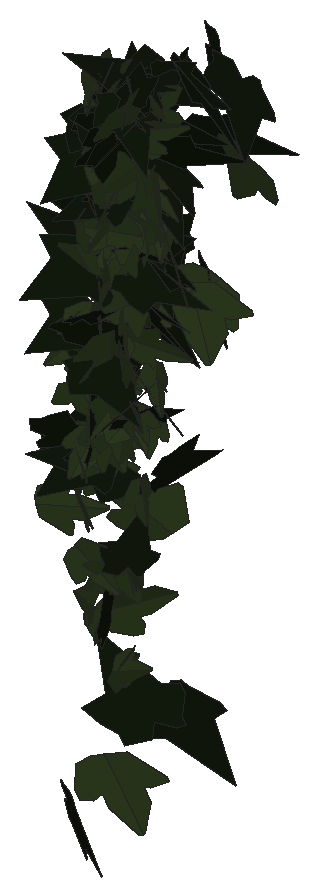
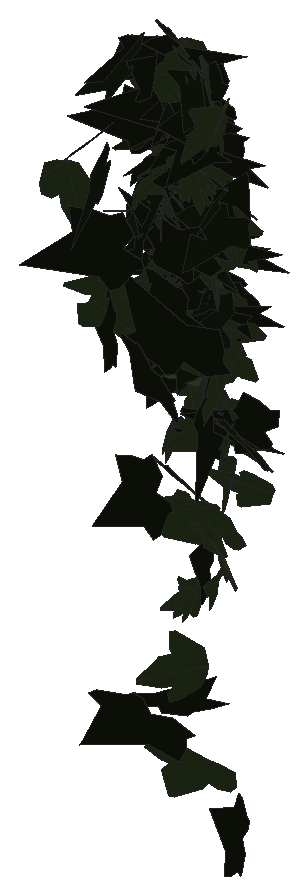
# SketchUp Ruby script. Lengths in inches.
U = 1.inch
M = Sketchup.active_model
def pt(a) = Geom::Point3d.new(a.map { |v| v * U })
def face(e, loops, mat)
  f = e.add_face(loops[0].map { |a| pt(a) })
  loops[1..].each { |l| e.add_face(l.map { |a| pt(a) }).erase! }
  f.material = f.back_material = mat if mat
  f
end
# faces: each face lists its corners as indices into pts; further lists are holes
def faces(e, pts, list, mat = nil) = list.each { |f| face(e, (f[0].is_a?(Array) ? f : [f]).map { |l| l.map { |i| pts[i] } }, mat) }
# xy, xz, yz: faces in a plane at the given z, y or x. An outline is a flat list of corners, or four numbers for a rectangle; further outlines are holes
def ring(l) = l.size == 4 ? [[l[0], l[1]], [l[2], l[1]], [l[2], l[3]], [l[0], l[3]]] : l.each_slice(2).to_a
def flat(e, list, mat, &to3) = list.each { |f| face(e, (f[0].is_a?(Array) ? f : [f]).map { |l| ring(l).map { |u, v| to3.(u, v) } }, mat) }
def xy(e, z, list, mat = nil) = flat(e, list, mat) { |x, y| [x, y, z] }
def xz(e, y, list, mat = nil) = flat(e, list, mat) { |x, z| [x, y, z] }
def yz(e, x, list, mat = nil) = flat(e, list, mat) { |y, z| [x, y, z] }
def lines(e, pts, list) = list.each { |a, b| e.add_line(pt(pts[a]), pt(pts[b])) }
# prism: a flat outline (further loops are holes) pulled along v
def prism(e, loops, v, mat = nil)
  f = face(e, loops, mat); d = Geom::Vector3d.new(v.map { |x| x * U })
  f.pushpull(f.normal.samedirection?(d) ? d.length : -d.length)
end
def box(e, o, s, mat = nil) = prism(e, [[o, [o[0] + s[0], o[1], o[2]], [o[0] + s[0], o[1] + s[1], o[2]], [o[0], o[1] + s[1], o[2]]]], [0, 0, s[2]], mat)
def at(x, y, z, deg = 0) = Geom::Transformation.translation(pt([x, y, z])) * Geom::Transformation.rotation(ORIGIN, Z_AXIS, deg.degrees)
def axes(o, x, y, z) = Geom::Transformation.new([*x, 0, *y, 0, *z, 0, *pt(o).to_a, 1])
def part(name) = M.definitions.add(name)
# library, detail: a bought-in or finely detailed component or shape, given as its bounding box
def library(name, o, s) = part(name).tap { |d| box(d.entities, o, s) }
def detail(e, o, s) = box(e.add_group.entities, o, s)
def put(e, d, t, mat = nil) = e.add_instance(d, t).tap { |i| i.material = mat if mat }
def group(e, t, mat = nil) = e.add_group.tap { |g| g.transformation = t; g.material = mat if mat }.entities
root = M.entities
M.materials.add("1026 AP 7946 SUNNY SIDE UP").color = [254, 231, 186]
M.materials.add("efeu1").color = [18, 25, 13]
M.materials.add("efeu2").color = [43, 57, 29]
c1 = part("ivyleaf_10")
p = [[0,0.5,-0.03],[-0.0625,2.02,-0.43],[-0.19,2.01,-0.46],[-0.54,1.05,-0.29],[-0.52,0.625,-0.18],[-0.83,0.76,-0.28],
  [-1.16,0.64,-0.33],[-1.15,0.33,-0.24],[-0.77,-0.39,0.02],[-0.3,-0.51,0.16],[0.04,-0.48,0.23],[-0.02,2.01,-0.4375],
  [-0.06,2.01,-0.43],[0.04,-0.49,0.23],[0.67,-0.49,0.14],[1.38,0.36,-0.2],[1.375,0.51,-0.24],[0.81,0.65,-0.19],
  [0.62,0.59,-0.15],[0.6,1.09,-0.28],[0.5,1.23,-0.31]]
faces(c1.entities,p,[[0,1,2,3,4,5,6,7,8,9,10],[11,12,0,13,14,15,16,17,18,19,20]],"efeu2")
c2 = part("ivyleaf_9")
p = [[1.54,2.16,1.25],[1.36,2.04,1.19],[-0.21,0.99,0.68],[-0.71,1.11,0.82],[-0.85,0.86,0.67],[-0.8,0.17,0.21],
  [-0.9,-0.01,0.1],[-0.67,-0.16,-0.02],[-0.08,-0.08,-0.05],[-0.03,-0.6,-0.4],[0.65,-0.88,-0.66],[0.83,-0.6,-0.49],
  [1.29,-0.42,-0.43],[1.8125,-0.07,-0.26],[1.21,0.44,0.15]]
faces(c2.entities,p,[[0,1,2,3,4,5,6,7,8,9,10,11,12,13,14]],"efeu1")
put(root,c1,axes([138.06,210.26,263.38],[0.1291,0.1731,-0.15782],[-0.14397,-0.12604,-0.19675],[-0.33485,0.12093,0.02375]),"1026 AP 7946 SUNNY SIDE UP")
put(root,c1,axes([137.23,210.13,261.82],[0.09734,-0.04348,-0.24254],[0.37472,0.03179,0.05875],[0.03186,-0.24111,0.05]),"1026 AP 7946 SUNNY SIDE UP")
put(root,c1,axes([138.36,210.2,263.44],[-0.32079,0.0153,-0.08144],[0.11047,-0.07182,-0.20131],[-0.06213,-0.2067,0.06255]),"1026 AP 7946 SUNNY SIDE UP")
put(root,c1,axes([138.26,210.23,265.55],[0.316,-0.15134,0.01152],[-0.00357,-0.02297,-0.25851],[0.23869,0.20001,-0.01912]),"1026 AP 7946 SUNNY SIDE UP")
put(root,c1,axes([137.63,210.17,263.5],[-0.23237,-0.14034,-0.09498],[0.17288,0.01065,-0.19993],[0.19866,-0.17343,0.06289]),"1026 AP 7946 SUNNY SIDE UP")
put(root,c2,axes([137.8,210.15,264.41],[0.16591,0.16497,-0.14641],[-0.09865,-0.12928,-0.20201],[-0.32886,0.12201,-0.01327]),"1026 AP 7946 SUNNY SIDE UP")
put(root,c2,axes([138.24,210.26,267.47],[0.00262,-0.25337,-0.06246],[0.00721,0.05921,-0.26063],[0.40906,0.00058,0.005]),"1026 AP 7946 SUNNY SIDE UP")
put(root,c1,axes([138.39,210.18,266.7],[-0.31364,0.01889,0.14931],[-0.22955,-0.03335,-0.20284],[0.00709,-0.24423,0.03778]),"1026 AP 7946 SUNNY SIDE UP")
put(root,c2,axes([137.88,210.22,263.87],[-0.03443,-0.1949,-0.15408],[0.17512,0.12485,-0.18504],[0.34315,-0.08327,0.07897]),"1026 AP 7946 SUNNY SIDE UP")
put(root,c1,axes([138.36,210.12,267.53],[-0.09058,-0.29287,-0.1462],[0.06632,0.13448,-0.30637],[0.50626,-0.07002,0.01398]),"1026 AP 7946 SUNNY SIDE UP")
put(root,c2,axes([137.79,210.29,262.58],[-0.42238,0.00458,-0.0159],[0.0235,-0.02618,-0.27564],[-0.00953,-0.26779,0.0251]),"1026 AP 7946 SUNNY SIDE UP")
put(root,c1,axes([137.73,210.27,262.8],[0.19876,0.17393,-0.1307],[-0.11112,-0.10666,-0.22208],[-0.32073,0.14474,-0.00405]),"1026 AP 7946 SUNNY SIDE UP")
put(root,c1,axes([138,210.2,262.97],[-0.30622,-0.07233,-0.06685],[0.11611,-0.01707,-0.21014],[0.09865,-0.20443,0.03984]),"1026 AP 7946 SUNNY SIDE UP")
put(root,c1,axes([138.31,210.06,259.99],[-0.02923,-0.06515,-0.21105],[0.14664,0.18242,-0.06754],[0.30396,-0.09427,0.01229]),"1026 AP 7946 SUNNY SIDE UP")
put(root,c2,axes([138.36,209.96,263.46],[0.0629,0.24625,0.17947],[0.05374,0.16948,-0.25596],[-0.46998,0.05234,-0.00525]),"1026 AP 7946 SUNNY SIDE UP")
put(root,c2,axes([137.6875,210.39,265.08],[-0.35934,-0.13219,0.12933],[-0.15226,-0.08395,-0.27154],[0.24383,-0.24724,0.02103]),"1026 AP 7946 SUNNY SIDE UP")
put(root,c2,axes([138.44,210.07,261.45],[-0.30501,0.14579,0.00188],[0.01738,0.01306,0.24944],[0.22858,0.19354,-0.01646]),"1026 AP 7946 SUNNY SIDE UP")
put(root,c1,axes([138.07,210.1,265.15],[0.08744,-0.14076,-0.18635],[-0.08457,0.17208,-0.15466],[0.34931,0.0769,0.0092]),"1026 AP 7946 SUNNY SIDE UP")
put(root,c1,axes([137.52,210.375,264.11],[0.14013,0.12261,-0.23008],[-0.17599,-0.19453,-0.15668],[-0.36096,0.14245,-0.01293]),"1026 AP 7946 SUNNY SIDE UP")
put(root,c2,axes([138.46,210.15,265.32],[0.2387,-0.13379,-0.13768],[0.12168,0.19977,-0.11496],[0.27039,0.02821,0.17328]),"1026 AP 7946 SUNNY SIDE UP")
put(root,c1,axes([137.59,210.26,261.19],[0.17176,0.02457,0.22149],[0.34002,-0.0098,-0.11216],[-0.00368,0.24083,-0.02574]),"1026 AP 7946 SUNNY SIDE UP")
put(root,c1,axes([138.2,210.41,263.17],[-0.37584,-0.01107,0.01569],[0.01872,-0.23912,0.01198],[0.02303,0.01371,0.24622]),"1026 AP 7946 SUNNY SIDE UP")
put(root,c1,axes([138,210.25,266.15],[0.13435,-0.22315,-0.02969],[-0.02544,0.02329,-0.24593],[0.35262,0.0867,-0.00643]),"1026 AP 7946 SUNNY SIDE UP")
put(root,c1,axes([137.85,210.11,260.6875],[0.00583,0.09087,0.22719],[-0.30492,0.12877,-0.05067],[-0.21708,-0.17844,0.07728]),"1026 AP 7946 SUNNY SIDE UP")
put(root,c2,axes([137.7,210.43,263.51],[0.03949,-0.03741,-0.27942],[0.3284,-0.17319,0.04355],[-0.2779,-0.20998,0.01176]),"1026 AP 7946 SUNNY SIDE UP")
put(root,c2,axes([137.56,210.42,264.28],[-0.29835,-0.13703,0.12554],[-0.13617,-0.08887,-0.24085],[0.2551,-0.20771,0.01826]),"1026 AP 7946 SUNNY SIDE UP")
put(root,c2,axes([137.93,210.24,264.5625],[-0.03994,0.20176,-0.15039],[-0.06662,-0.14923,-0.20415],[-0.38695,0.00487,0.05067]),"1026 AP 7946 SUNNY SIDE UP")
put(root,c2,axes([138.08,210.34,262.57],[-0.11334,-0.0979,-0.25865],[-0.28731,-0.17249,0.1226],[-0.31034,0.19544,-0.01904]),"1026 AP 7946 SUNNY SIDE UP")
put(root,c1,axes([138.27,210.2,264.12],[-0.23443,0.15909,0.05273],[-0.09369,0.01221,-0.22176],[-0.24504,-0.15687,0.03434]),"1026 AP 7946 SUNNY SIDE UP")
put(root,c1,axes([137.89,210.39,264.03],[-0.08853,0.14987,-0.2013],[-0.12789,-0.20131,-0.13552],[-0.36661,0.03404,0.09588]),"1026 AP 7946 SUNNY SIDE UP")
put(root,c1,axes([138.36,210.23,263.46],[-0.20682,0.17572,0.00459],[-0.03538,-0.01255,-0.22466],[-0.27409,-0.13098,0.02553]),"1026 AP 7946 SUNNY SIDE UP")
put(root,c1,axes([137.85,210.23,262.84],[0.24639,-0.1083,-0.13648],[-0.16618,0.07895,-0.19573],[0.21065,0.18897,0.00522]),"1026 AP 7946 SUNNY SIDE UP")
put(root,c1,axes([138.49,210.41,263.3],[-0.1745,-0.15199,0.13368],[0.1688,-0.17117,-0.11222],[0.2661,0.00891,0.15885]),"1026 AP 7946 SUNNY SIDE UP")
put(root,c1,axes([138.16,210.25,261.13],[0.27295,0.05037,-0.14511],[-0.23495,0.04165,-0.17376],[-0.01802,0.21982,0.06758]),"1026 AP 7946 SUNNY SIDE UP")
put(root,c1,axes([138.15,210.26,263.04],[0.31119,-0.13128,-0.02731],[0.00583,0.05136,-0.24001],[0.21028,0.19285,0.04706]),"1026 AP 7946 SUNNY SIDE UP")
put(root,c1,axes([138.26,210.27,265.76],[0.13153,-0.04834,-0.2422],[-0.35967,0.05844,-0.09599],[0.11296,0.24234,-0.02361]),"1026 AP 7946 SUNNY SIDE UP")
put(root,c2,axes([138.01,209.98,266.98],[0.16347,0.16635,0.31777],[0.30824,0.23791,-0.19947],[-0.45521,0.22084,-0.02095]),"1026 AP 7946 SUNNY SIDE UP")
put(root,c1,axes([137.94,210.23,262.45],[-0.20537,-0.11251,-0.17863],[0.271,0.05264,-0.16925],[0.1779,-0.21008,0.0516]),"1026 AP 7946 SUNNY SIDE UP")
put(root,c1,axes([137.61,210.2,262.01],[-0.21876,0.19758,0.08419],[-0.09123,0.05757,-0.24821],[-0.32289,-0.15012,0.01309]),"1026 AP 7946 SUNNY SIDE UP")
put(root,c1,axes([138.3,210.28,264.84],[0.27935,-0.10012,-0.15345],[-0.21994,0.05282,-0.20893],[0.17565,0.22537,-0.01756]),"1026 AP 7946 SUNNY SIDE UP")
put(root,c1,axes([137.98,210.27,264.24],[-0.12535,-0.27978,-0.05718],[0.05056,0.04679,-0.29886],[0.44515,-0.0841,0.01784]),"1026 AP 7946 SUNNY SIDE UP")
put(root,c1,axes([138.01,210.41,265.78],[0.05977,0.13956,-0.19016],[-0.1365,-0.16565,-0.14778],[-0.33836,0.09148,0.02603]),"1026 AP 7946 SUNNY SIDE UP")
put(root,c1,axes([138.23,210.34,264.57],[0.0147,0.20836,-0.09113],[-0.00596,-0.08957,-0.21539],[-0.35661,0.01009,-0.00016]),"1026 AP 7946 SUNNY SIDE UP")
put(root,c2,axes([137.16,210.18,262.7],[0.1558,0.02753,0.23136],[0.34623,0.04394,-0.10545],[-0.0808,0.24136,-0.00572]),"1026 AP 7946 SUNNY SIDE UP")
put(root,c2,axes([138.08,210.37,265.1],[-0.21253,0.14962,-0.15852],[0.10289,-0.14549,-0.20468],[-0.32242,-0.14506,0.03918]),"1026 AP 7946 SUNNY SIDE UP")
put(root,c1,axes([137.57,210.23,264.31],[0.09253,-0.00735,-0.22715],[0.33398,0.06343,0.0566],[0.09355,-0.21918,0.02261]),"1026 AP 7946 SUNNY SIDE UP")
put(root,c1,axes([138.31,210.14,259.94],[0.04389,0.00482,0.22162],[-0.12511,0.20175,0.00716],[-0.31432,-0.07963,0.02809]),"1026 AP 7946 SUNNY SIDE UP")
put(root,c2,axes([138.19,210.0625,267.12],[0.00377,0.01178,-0.34694],[-0.23955,0.30051,0.01146],[0.47274,0.15218,0.00857]),"1026 AP 7946 SUNNY SIDE UP")
put(root,c1,axes([138.29,210.26,261.32],[-0.23422,0.15956,0.04043],[-0.0561,0.01905,-0.22437],[-0.25186,-0.15263,0.01238]),"1026 AP 7946 SUNNY SIDE UP")
put(root,c1,axes([137.54,210.3,265.23],[-0.34733,-0.02559,-0.07688],[0.12022,-0.01652,-0.22785],[0.02969,-0.23252,0.02326]),"1026 AP 7946 SUNNY SIDE UP")
put(root,c1,axes([137.58,210.25,262.59],[-0.14894,0.23669,0.05032],[-0.04254,0.0403,-0.2622],[-0.37721,-0.098,0.0097]),"1026 AP 7946 SUNNY SIDE UP")
put(root,c1,axes([138.32,210.2,266.6],[0.0605,-0.07099,-0.25152],[-0.24636,0.18734,-0.08059],[0.3141,0.16061,-0.01477]),"1026 AP 7946 SUNNY SIDE UP")
put(root,c1,axes([138.14,210.36,265.79],[0.35493,-0.06052,-0.03092],[-0.052,-0.00908,-0.24016],[0.09235,0.22749,-0.01638]),"1026 AP 7946 SUNNY SIDE UP")
put(root,c2,axes([138.3125,210.32,264.875],[0.36618,-0.09698,0.01833],[0.01316,-0.02743,-0.25905],[0.15464,0.23198,-0.02136]),"1026 AP 7946 SUNNY SIDE UP")
put(root,c1,axes([138.38,210.37,262.35],[0.01363,-0.22637,0.02295],[0.13255,-0.01871,-0.21723],[0.33242,0.01674,0.08568]),"1026 AP 7946 SUNNY SIDE UP")
put(root,c1,axes([138.55,210.33,266.5],[0.04211,-0.27743,-0.04055],[0.13704,0.04433,-0.27143],[0.41838,0.0134,0.09299]),"1026 AP 7946 SUNNY SIDE UP")
put(root,c2,axes([138.03,210.11,260.43],[-0.00106,-0.03669,0.34532],[0.15039,0.32163,0.03832],[-0.50878,0.09515,0.01061]),"1026 AP 7946 SUNNY SIDE UP")
put(root,c1,axes([138.29,210.25,267.63],[0.12789,-0.1941,-0.14445],[-0.00913,0.14531,-0.21151],[0.37538,0.06966,0.04407]),"1026 AP 7946 SUNNY SIDE UP")
put(root,c1,axes([138.5625,210.41,263.93],[-0.01304,-0.22331,0.06904],[0.17469,-0.06387,-0.20166],[0.32296,0.02553,0.11186]),"1026 AP 7946 SUNNY SIDE UP")
put(root,c2,axes([138.13,210.42,264.86],[0.17381,-0.14455,0.18425],[0.2437,-0.10096,-0.1825],[0.26848,0.18522,0.04638]),"1026 AP 7946 SUNNY SIDE UP")
put(root,c1,axes([137.83,210.1875,260.33],[0.01212,0.07937,-0.21081],[0.01098,0.20502,0.08321],[0.34561,-0.0093,0.00475]),"1026 AP 7946 SUNNY SIDE UP")
put(root,c2,axes([137.69,210.51,266.46],[-0.38029,-0.12053,0.04958],[-0.05266,-0.04187,-0.27769],[0.19758,-0.24315,0.02143]),"1026 AP 7946 SUNNY SIDE UP")
put(root,c2,axes([138.01,210.41,266.17],[-0.39593,0.07153,0.00373],[-0.01452,-0.0208,-0.26879],[-0.11165,-0.25096,0.02174]),"1026 AP 7946 SUNNY SIDE UP")
put(root,c1,axes([137.68,210.45,264.8],[-0.1059,0.19768,-0.17616],[0.05238,-0.16981,-0.21534],[-0.4088,-0.07297,0.01804]),"1026 AP 7946 SUNNY SIDE UP")
put(root,c1,axes([137.74,210.34,263.42],[-0.05328,0.25717,-0.01885],[-0.00322,-0.0202,-0.2673],[-0.40556,-0.03363,0.0046]),"1026 AP 7946 SUNNY SIDE UP")
put(root,c2,axes([138.38,210.17,267.62],[-0.32567,0.14063,-0.1387],[-0.16076,0.09009,0.25797],[0.26155,0.23048,-0.01415]),"1026 AP 7946 SUNNY SIDE UP")
put(root,c1,axes([138.17,210.39,265.39],[0.34016,0.07934,0.03953],[0.06434,-0.00169,-0.23685],[-0.12239,0.21962,-0.01465]),"1026 AP 7946 SUNNY SIDE UP")
put(root,c2,axes([138.41,210.22,263.34],[0.20857,0.21802,0.05732],[0.06092,0.04004,-0.26238],[-0.34803,0.13767,-0.01157]),"1026 AP 7946 SUNNY SIDE UP")
put(root,c1,axes([138.41,210.3125,264.31],[0.06889,-0.01548,0.22669],[0.27726,0.1374,-0.02539],[-0.20863,0.17748,0.0411]),"1026 AP 7946 SUNNY SIDE UP")
put(root,c1,axes([137.83,210.46,266.93],[-0.09931,0.20253,-0.1201],[0.0343,-0.11632,-0.21888],[-0.36676,-0.06572,0.01205]),"1026 AP 7946 SUNNY SIDE UP")
put(root,c1,axes([138.26,210.51,265.72],[0.28664,-0.10388,0.13159],[0.15876,-0.08109,-0.21588],[0.20539,0.20766,-0.01677]),"1026 AP 7946 SUNNY SIDE UP")
put(root,c2,axes([138.19,210.16,266.98],[-0.15929,0.16339,-0.26219],[-0.20248,0.22064,0.1993],[0.43165,0.16379,-0.00327]),"1026 AP 7946 SUNNY SIDE UP")
put(root,c1,axes([138.26,210.35,267.0625],[-0.11668,-0.11329,0.23022],[0.26138,0.15301,0.13728],[-0.29598,0.17978,0.03047]),"1026 AP 7946 SUNNY SIDE UP")
put(root,c1,axes([137.6,210.33,263.8],[0.1366,0.10626,0.23449],[0.27412,0.14702,-0.13876],[-0.28319,0.19357,-0.02121]),"1026 AP 7946 SUNNY SIDE UP")
put(root,c1,axes([138,210.4375,266.8],[-0.35541,-0.11411,-0.08446],[0.15781,-0.02408,-0.25264],[0.15378,-0.23901,0.06405]),"1026 AP 7946 SUNNY SIDE UP")
put(root,c2,axes([137.27,210.29,262.52],[-0.24755,0.21408,-0.00236],[0.01465,0.0112,0.27344],[0.33635,0.15707,-0.01365]),"1026 AP 7946 SUNNY SIDE UP")
put(root,c2,axes([138.2,210.48,263.76],[0.29697,-0.15187,0.02945],[0.01264,-0.03678,-0.24871],[0.24292,0.18758,-0.02306]),"1026 AP 7946 SUNNY SIDE UP")
put(root,c1,axes([138.21,210.39,266.36],[-0.27886,-0.13633,-0.1925],[0.28353,0.06447,-0.22531],[0.22622,-0.24884,0.0451]),"1026 AP 7946 SUNNY SIDE UP")
put(root,c1,axes([137.62,210.28,265.66],[0.00892,0.1432,0.21459],[-0.10851,0.2005,-0.13943],[-0.38128,-0.05371,0.0447]),"1026 AP 7946 SUNNY SIDE UP")
put(root,c2,axes([137.65,210.59,267.35],[0.12685,-0.13472,0.21145],[0.15801,-0.17989,-0.16278],[0.35334,0.12881,-0.00312]),"1026 AP 7946 SUNNY SIDE UP")
put(root,c2,axes([138.51,210.65,265.3],[-0.10666,-0.17304,0.16589],[0.154,-0.17392,-0.15014],[0.33943,0.02453,0.12025]),"1026 AP 7946 SUNNY SIDE UP")
put(root,c2,axes([137.72,210.44,265.18],[-0.06588,0.10834,0.25322],[-0.38762,0.08189,-0.0802],[-0.16554,-0.23487,0.08701]),"1026 AP 7946 SUNNY SIDE UP")
put(root,c2,axes([138.08,210.39,266.09],[0.2858,0.15942,-0.10624],[-0.11329,-0.07553,-0.24935],[-0.27706,0.19533,-0.00763]),"1026 AP 7946 SUNNY SIDE UP")
put(root,c1,axes([137.81,210.33,264.89],[0.06337,-0.16656,-0.25008],[-0.12485,0.22879,-0.17465],[0.44448,0.08802,-0.0134]),"1026 AP 7946 SUNNY SIDE UP")
put(root,c2,axes([138.08,210.35,265.35],[0.36472,0.07165,0.09108],[0.12948,0.03153,-0.24984],[-0.12278,0.24607,0.00708]),"1026 AP 7946 SUNNY SIDE UP")
put(root,c1,axes([137.91,210.53,265.88],[0.39798,0.02332,-0.08058],[-0.12016,-0.02307,-0.26152],[-0.04566,0.26395,-0.01417]),"1026 AP 7946 SUNNY SIDE UP")
put(root,c2,axes([137.97,210.39,264.24],[0.3104,0.02193,0.1639],[0.24927,0.01249,-0.20451],[-0.03919,0.25315,-0.00261]),"1026 AP 7946 SUNNY SIDE UP")
put(root,c2,axes([138.41,210.57,267.62],[-0.13426,0.03165,0.27067],[-0.41541,-0.0226,-0.08584],[0.01868,-0.27516,0.03654]),"1026 AP 7946 SUNNY SIDE UP")
put(root,c1,axes([138.4,210.45,265.73],[0.06492,-0.03385,-0.27191],[-0.37944,0.10735,-0.05248],[0.17564,0.24442,-0.01288]),"1026 AP 7946 SUNNY SIDE UP")
put(root,c1,axes([138.32,210.47,265.9375],[-0.32498,0.10555,0.03937],[-0.06917,-0.00384,-0.23791],[-0.16204,-0.21004,0.02259]),"1026 AP 7946 SUNNY SIDE UP")
put(root,c2,axes([138.32,210.55,265.4],[0.0695,-0.2278,-0.08711],[-0.03778,0.0801,-0.23845],[0.3795,0.04969,-0.00779]),"1026 AP 7946 SUNNY SIDE UP")
put(root,c1,axes([137.73,210.33,263.0625],[-0.04021,0.11801,0.24519],[-0.14572,0.2194,-0.12139],[-0.39046,-0.09403,0.02005]),"1026 AP 7946 SUNNY SIDE UP")
put(root,c2,axes([137.56,210.48,264.26],[0.02953,-0.184,-0.2067],[0.03669,0.20042,-0.18691],[0.42527,-0.00452,0.03048]),"1026 AP 7946 SUNNY SIDE UP")
put(root,c1,axes([138.48,210.56,264.76],[0.08815,-0.24132,0.01013],[-0.00106,-0.01166,-0.25527],[0.37985,0.05597,-0.00306]),"1026 AP 7946 SUNNY SIDE UP")
put(root,c1,axes([137.86,210.25,266.4],[0.07647,0.04952,-0.36506],[0.17641,0.33777,0.06642],[0.5347,-0.11852,0.0303]),"1026 AP 7946 SUNNY SIDE UP")
put(root,c2,axes([137.51,210.5625,265.61],[0.29645,-0.03204,0.19977],[-0.27657,0.09297,0.19236],[-0.13856,-0.25412,0.04348]),"1026 AP 7946 SUNNY SIDE UP")
put(root,c1,axes([137.48,210.53,265.72],[-0.40355,-0.01928,0.1011],[-0.14934,-0.03867,-0.26363],[0.04981,-0.27207,0.02867]),"1026 AP 7946 SUNNY SIDE UP")
put(root,c1,axes([137.75,210.52,267.7],[0.1489,-0.24335,-0.07984],[-0.0253,0.07533,-0.26829],[0.40013,0.09532,0.01275]),"1026 AP 7946 SUNNY SIDE UP")
put(root,c1,axes([138.13,210.75,267.625],[0.08301,0.09054,-0.29585],[-0.19595,-0.25942,-0.10918],[-0.43187,0.13511,-0.00733]),"1026 AP 7946 SUNNY SIDE UP")
put(root,c1,axes([138.53,210.7,265.875],[-0.10821,-0.1763,0.16759],[0.15626,-0.17587,-0.15314],[0.34448,0.02439,0.12211]),"1026 AP 7946 SUNNY SIDE UP")
put(root,c1,axes([137.81,210.58,266.2],[-0.11311,-0.25865,0.01499],[0.00388,-0.0173,-0.27658],[0.40746,-0.07164,0.00679]),"1026 AP 7946 SUNNY SIDE UP")
put(root,c1,axes([138.2,210.57,267.48],[-0.31471,0.12751,-0.06115],[0.05865,-0.05271,-0.24357],[-0.21373,-0.20221,0.0232]),"1026 AP 7946 SUNNY SIDE UP")
put(root,c1,axes([137.44,210.41,263.66],[0.04574,0.09576,-0.24281],[0.08558,0.22995,0.10428],[0.39157,-0.06145,0.00557]),"1026 AP 7946 SUNNY SIDE UP")
put(root,c2,axes([138.45,210.76,266.59],[0.01497,-0.24025,0.088],[0.15112,-0.0771,-0.23118],[0.37215,0.04097,0.09033]),"1026 AP 7946 SUNNY SIDE UP")
put(root,c1,axes([137.79,210.625,266.68],[0.06581,0.2654,-0.04202],[-0.00669,-0.04214,-0.27702],[-0.42252,0.04201,-0.00216]),"1026 AP 7946 SUNNY SIDE UP")
put(root,c2,axes([137.5,210.63,265.95],[0.27662,-0.21677,-0.08895],[-0.10083,0.05746,-0.28695],[0.35202,0.18679,-0.01229]),"1026 AP 7946 SUNNY SIDE UP")
put(root,c2,axes([138.32,210.56,265.4],[-0.21879,0.15116,0.14317],[-0.17027,0.0874,-0.21042],[-0.27324,-0.1755,0.01648]),"1026 AP 7946 SUNNY SIDE UP")
put(root,c2,axes([136.96,210.82,257.34],[0.13642,-0.05563,-0.33629],[0.48921,-0.10092,0.10241],[-0.17688,-0.32202,0.02388]),"1026 AP 7946 SUNNY SIDE UP")
put(root,c1,axes([138.23,210.64,267.29],[-0.30342,-0.09253,0.1414],[0.18361,0.07446,0.22043],[-0.18545,0.22511,-0.01311]),"1026 AP 7946 SUNNY SIDE UP")
put(root,c1,axes([138.32,210.52,264.89],[-0.05588,-0.09937,-0.22633],[0.13344,0.2021,-0.10741],[0.35402,-0.09186,0.00476]),"1026 AP 7946 SUNNY SIDE UP")
put(root,c2,axes([138.34,210.73,266.37],[0.05533,-0.25901,-0.07294],[-0.021,0.06814,-0.26886],[0.42109,0.03743,-0.00382]),"1026 AP 7946 SUNNY SIDE UP")
put(root,c2,axes([138.08,210.47,263.75],[-0.05264,0.15802,0.24219],[-0.08793,0.22747,-0.16502],[-0.43545,-0.06504,0.00404]),"1026 AP 7946 SUNNY SIDE UP")
put(root,c2,axes([137.87,210.46,267.4375],[0.08211,0.22309,0.14909],[0.03371,0.14218,-0.23499],[-0.41568,0.0556,0.01039]),"1026 AP 7946 SUNNY SIDE UP")
put(root,c2,axes([137.79,210.49,267.13],[0.13105,0.11562,-0.35246],[0.26145,0.30017,0.14771],[0.50519,-0.18534,0.01499]),"1026 AP 7946 SUNNY SIDE UP")
put(root,c2,axes([137.7,210.46,262.82],[0.01251,-0.05652,-0.38347],[-0.42926,0.25507,-0.04445],[0.40696,0.27078,-0.0351]),"1026 AP 7946 SUNNY SIDE UP")
put(root,c2,axes([138.8,210.61,265.12],[0.00744,-0.1944,0.32854],[-0.02596,0.31962,0.20214],[-0.58818,-0.01656,-0.00476]),"1026 AP 7946 SUNNY SIDE UP")
put(root,c2,axes([137.33,210.79,264.34],[0.44832,-0.23306,0.03843],[0.01993,-0.04537,-0.37862],[0.37093,0.28412,-0.02611]),"1026 AP 7946 SUNNY SIDE UP")
put(root,c1,axes([137.64,210.74,258.09],[0.43204,0.14088,0.15572],[0.23305,0.03897,-0.3164],[-0.22507,0.31078,-0.0287]),"1026 AP 7946 SUNNY SIDE UP")
put(root,c2,axes([137.6,210.68,267.01],[0.02889,-0.14131,-0.25967],[0.01021,0.25191,-0.14399],[0.45316,0.00333,0.0198]),"1026 AP 7946 SUNNY SIDE UP")
put(root,c2,axes([138.43,210.61,267.375],[-0.05924,-0.03424,0.27581],[0.23549,0.22247,0.05229],[-0.35343,0.15397,-0.01139]),"1026 AP 7946 SUNNY SIDE UP")
put(root,c1,axes([138.29,210.59,265.59],[0.02996,0.05477,-0.26075],[-0.01974,0.25399,0.05707],[0.40719,0.00828,0.02195]),"1026 AP 7946 SUNNY SIDE UP")
put(root,c2,axes([137.48,210.74,266.89],[-0.02208,-0.19795,-0.23253],[0.01837,0.22431,-0.20311],[0.47038,-0.01805,-0.00298]),"1026 AP 7946 SUNNY SIDE UP")
put(root,c2,axes([138.46,210.68,266.74],[0.23722,0.02724,0.21531],[0.31822,0.0524,-0.15734],[-0.09172,0.25225,0.011]),"1026 AP 7946 SUNNY SIDE UP")
put(root,c2,axes([138.4,210.64,267.74],[0.03841,-0.00526,-0.282],[0.04669,0.27322,-0.00108],[0.42791,-0.02934,0.02543]),"1026 AP 7946 SUNNY SIDE UP")
put(root,c2,axes([137.72,210.86,265.13],[-0.02797,0.04917,0.33529],[0.36601,-0.22819,0.04733],[0.36534,0.23237,-0.02174]),"1026 AP 7946 SUNNY SIDE UP")
put(root,c1,axes([137.39,210.62,267.18],[0.03291,-0.0137,-0.29694],[-0.03421,0.28802,-0.01405],[0.45232,0.02278,0.02054]),"1026 AP 7946 SUNNY SIDE UP")
put(root,c2,axes([137.3,210.68,265.82],[0.40152,0.0681,-0.09225],[-0.17028,0.08566,-0.24945],[-0.04968,0.25682,0.10944]),"1026 AP 7946 SUNNY SIDE UP")
put(root,c2,axes([137.7,210.68,267],[-0.04488,0.20303,-0.16693],[-0.14281,0.1461,0.20449],[0.38388,0.07809,0.05656]),"1026 AP 7946 SUNNY SIDE UP")
put(root,c1,axes([137.46,210.71,267.12],[0.02175,0.15197,0.26598],[-0.05169,0.25681,-0.15292],[-0.46705,-0.02134,0.02931]),"1026 AP 7946 SUNNY SIDE UP")
put(root,c2,axes([138.08,210.95,258.87],[-0.43166,-0.19518,0.05298],[0.04512,0.05008,0.34643],[-0.31461,0.27498,-0.02301]),"1026 AP 7946 SUNNY SIDE UP")
put(root,c1,axes([138.12,211,261.54],[0.31004,0.10858,0.27031],[-0.39166,-0.08571,0.22941],[0.21254,-0.31632,0.02843]),"1026 AP 7946 SUNNY SIDE UP")
put(root,c2,axes([138.55,211.05,267.74],[0.32614,-0.25793,-0.0331],[-0.05491,0.0112,-0.34027],[0.40471,0.20937,-0.01949]),"1026 AP 7946 SUNNY SIDE UP")
put(root,c2,axes([137.625,211.1,264.58],[-0.00751,-0.06406,-0.38267],[0.58108,0.0706,-0.01704],[0.11392,-0.36435,0.0617]),"1026 AP 7946 SUNNY SIDE UP")
put(root,c1,axes([138.59,211.11,264.61],[0.39057,0.24004,0.05927],[0.09243,0.01977,-0.3547],[-0.37645,0.2539,-0.0256]),"1026 AP 7946 SUNNY SIDE UP")
put(root,c2,axes([138.01,211.33,258.92],[-0.13375,-0.11533,-0.32612],[0.36343,0.21665,-0.14433],[0.38412,-0.24514,0.023]),"1026 AP 7946 SUNNY SIDE UP")
put(root,c1,axes([138.44,211.54,264.54],[0.41238,0.0444,-0.20116],[-0.29028,-0.07208,-0.2724],[-0.12297,0.31908,-0.03155]),"1026 AP 7946 SUNNY SIDE UP")
put(root,c2,axes([137.99,211.23,261.99],[0.13639,0.19188,0.28565],[0.2392,0.23199,-0.2139],[-0.47161,0.17316,-0.02588]),"1026 AP 7946 SUNNY SIDE UP")
put(root,c1,axes([137.28,211.39,259.86],[0.05678,-0.03373,0.35089],[0.0306,0.34233,0.03478],[-0.53762,0.01593,0.03904]),"1026 AP 7946 SUNNY SIDE UP")
put(root,c2,axes([138.16,211.83,264.47],[0.06127,-0.05463,-0.33489],[0.48618,-0.10652,0.05606],[-0.17828,-0.30927,0.03777]),"1026 AP 7946 SUNNY SIDE UP")
put(root,c2,axes([137.1875,211.69,264.37],[-0.26625,0.03696,0.34556],[0.44476,-0.18872,0.16752],[0.2888,0.3247,0.0606]),"1026 AP 7946 SUNNY SIDE UP")
put(root,c1,axes([138.97,211.7,266.3],[-0.4277,0.10463,0.162],[-0.24546,0.02882,-0.29889],[-0.1658,-0.31256,0.02462]),"1026 AP 7946 SUNNY SIDE UP")
put(root,c2,axes([138.4375,212.2,267.03],[-0.00262,-0.31677,0.10355],[-0.01204,-0.10225,-0.32686],[0.52328,-0.00394,-0.00701]),"1026 AP 7946 SUNNY SIDE UP")
put(root,c2,axes([137.125,212.375,264.52],[-0.23922,-0.03671,-0.33181],[0.50851,-0.03837,-0.15318],[-0.03032,-0.35395,0.04891]),"1026 AP 7946 SUNNY SIDE UP")
put(root,c2,axes([137.68,212.31,266],[0.34097,0.12553,0.22413],[0.32675,0.07013,-0.25549],[-0.22014,0.29854,-0.03207]),"1026 AP 7946 SUNNY SIDE UP")
put(root,c2,axes([137.8,212.45,267.13],[0.32029,-0.17094,-0.25346],[-0.33179,0.12768,-0.2717],[0.33262,0.29197,-0.02696]),"1026 AP 7946 SUNNY SIDE UP")
